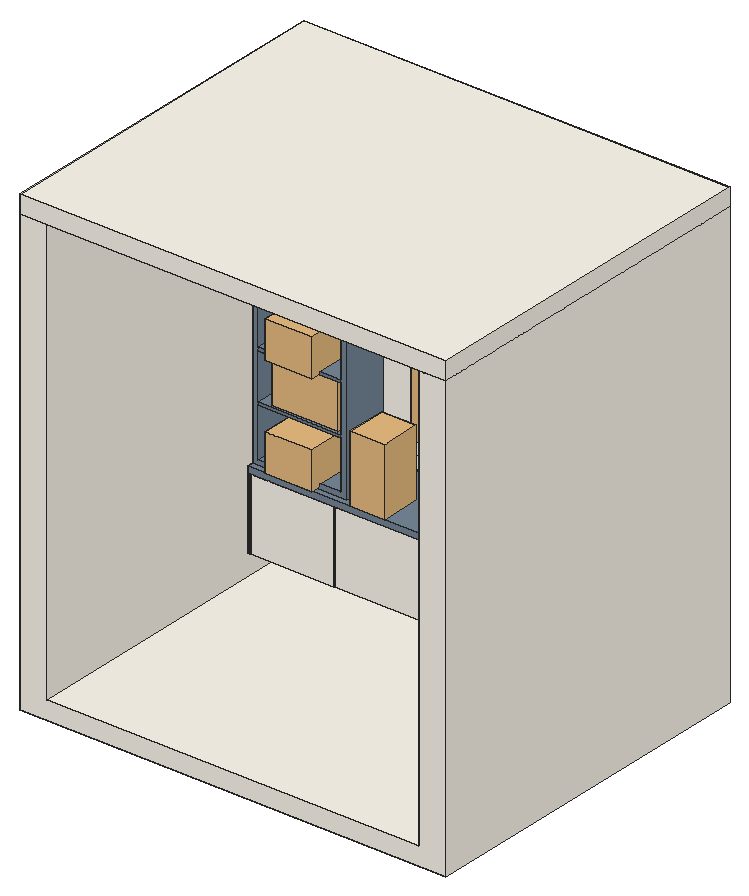
# SketchUp Ruby script. Lengths in inches.
U = 1.inch
M = Sketchup.active_model
def pt(a) = Geom::Point3d.new(a.map { |v| v * U })
def face(e, loops, mat)
  f = e.add_face(loops[0].map { |a| pt(a) })
  loops[1..].each { |l| e.add_face(l.map { |a| pt(a) }).erase! }
  f.material = f.back_material = mat if mat
  f
end
# faces: each face lists its corners as indices into pts; further lists are holes
def faces(e, pts, list, mat = nil) = list.each { |f| face(e, (f[0].is_a?(Array) ? f : [f]).map { |l| l.map { |i| pts[i] } }, mat) }
# xy, xz, yz: faces in a plane at the given z, y or x. An outline is a flat list of corners, or four numbers for a rectangle; further outlines are holes
def ring(l) = l.size == 4 ? [[l[0], l[1]], [l[2], l[1]], [l[2], l[3]], [l[0], l[3]]] : l.each_slice(2).to_a
def flat(e, list, mat, &to3) = list.each { |f| face(e, (f[0].is_a?(Array) ? f : [f]).map { |l| ring(l).map { |u, v| to3.(u, v) } }, mat) }
def xy(e, z, list, mat = nil) = flat(e, list, mat) { |x, y| [x, y, z] }
def xz(e, y, list, mat = nil) = flat(e, list, mat) { |x, z| [x, y, z] }
def yz(e, x, list, mat = nil) = flat(e, list, mat) { |y, z| [x, y, z] }
def lines(e, pts, list) = list.each { |a, b| e.add_line(pt(pts[a]), pt(pts[b])) }
# prism: a flat outline (further loops are holes) pulled along v
def prism(e, loops, v, mat = nil)
  f = face(e, loops, mat); d = Geom::Vector3d.new(v.map { |x| x * U })
  f.pushpull(f.normal.samedirection?(d) ? d.length : -d.length)
end
def box(e, o, s, mat = nil) = prism(e, [[o, [o[0] + s[0], o[1], o[2]], [o[0] + s[0], o[1] + s[1], o[2]], [o[0], o[1] + s[1], o[2]]]], [0, 0, s[2]], mat)
def at(x, y, z, deg = 0) = Geom::Transformation.translation(pt([x, y, z])) * Geom::Transformation.rotation(ORIGIN, Z_AXIS, deg.degrees)
def axes(o, x, y, z) = Geom::Transformation.new([*x, 0, *y, 0, *z, 0, *pt(o).to_a, 1])
def part(name) = M.definitions.add(name)
# library, detail: a bought-in or finely detailed component or shape, given as its bounding box
def library(name, o, s) = part(name).tap { |d| box(d.entities, o, s) }
def detail(e, o, s) = box(e.add_group.entities, o, s)
def put(e, d, t, mat = nil) = e.add_instance(d, t).tap { |i| i.material = mat if mat }
def group(e, t, mat = nil) = e.add_group.tap { |g| g.transformation = t; g.material = mat if mat }.entities
root = M.entities
M.materials.add("[0052_FloralWhite]").color = [255, 250, 240]
M.materials.add("[0110_LightSlateGray]").color = [119, 136, 153]
M.materials.add("[0111_SlateGray]").color = [112, 128, 144]
c1 = library("TV (1)",[0,0,0],[57.09,0.98,33.46])
c2 = library("Potted plant",[-1.15,-1.29,0],[7.65,7.78,5.89])
c3 = library("plants",[-0.26,-0.03,0],[11.57,13.37,22.79])
c4 = library("Decorative sailing ship",[0,0,0],[34.02,11.3,29.65])
c5 = library("horse",[-15.44,-5.1,-1.44],[29.35,10.2,27.55])
box(root,[0,0,150],[144,120,6],"[0052_FloralWhite]")
put(root,c1,axes([52.71,99.5,56.52],[1,0,0],[0,2.85,0],[0,0,1]))
put(root,c2,axes([18.09,86.57,40.3],[2.08,0,0],[0,2.0976,0],[0,0,2.12906]))
put(root,c2,axes([18.09,86.57,107],[2.08,0,0],[0,2.0976,0],[0,0,2.12906]))
put(root,c2,axes([18.09,86.57,74.48],[2.08,0,0],[0,2.0976,0],[0,0,2.12906]))
put(root,c2,axes([103.27,88.1875,113.32],[2.08,0,0],[0,2.0976,0],[0,0,2.12906]))
put(root,c2,axes([44.71,88.1875,113.32],[2.08,0,0],[0,2.0976,0],[0,0,2.12906]))
put(root,c3,at(43.99,85,39.5625))
put(root,c4,axes([10.82,82.23,91.875],[0.7885,0,0],[0,1.67,0],[0,0,0.5025]))
put(root,c5,axes([26.54,96.08,58.2],[0.7654,0,0],[0,1.59,0],[0,0,0.61717]))
g1 = group(root,at(0,0,0))
xy(g1,0,[[0,0,144,120]])
xy(g1,6,[[9,0,135,0,135,109,132.6,109,132.6,111,130.2,111,130.2,109,127.8,109,127.8,111,125.4,111,125.4,109,123,109,123,111,120.6,111,120.6,109,118.2,109,118.2,111,115.8,111,115.8,109,113.4,109,113.4,111,111,111,111,109,108.6,109,108.6,111,106.2,111,106.2,109,103.8,109,103.8,111,101.4,111,101.4,109,99,109,99,111,9,111]],"[0052_FloralWhite]")
xy(g1,13.1875,[[9,85,9,111,99,111,99,109,125.1875,109,125.1875,85,124.33,85,124.33,89.0625,124.13,89.0625,124.13,85,95.68,85,95.68,89.0625,95.48,89.0625,95.48,85,67.02,85,67.02,89.0625,66.82,89.0625,66.82,85,38.37,85,38.37,89.0625,38.17,89.0625,38.17,85,9.91,85,9.91,89.0625,9.71,89.0625,9.71,85]],"[0052_FloralWhite]")
xy(g1,37.36,[[9.91,85,38.17,85,38.17,89.0625,38.37,89.0625,38.37,85,66.82,85,66.82,89.0625,67.02,89.0625,67.02,85,95.48,85,95.48,89.0625,95.68,89.0625,95.68,85,124.13,85,124.13,89.0625,124.33,89.0625,124.33,90,9.71,90,9.71,89.0625,9.91,89.0625]])
xy(g1,37.5625,[[9.71,85,124.33,90]])
xy(g1,39.5625,[[9,85,125.1875,85,125.1875,109,99,109,99,111,40.875,111,40.875,87,9,87]],"[0110_LightSlateGray]")
xy(g1,41.1875,[[11,87,38.875,111]],"[0110_LightSlateGray]")
xy(g1,50.4375,[[40.875,102.3,125.1875,103.11]])
xy(g1,57.75,[[11,87,38.875,111]],"[0110_LightSlateGray]")
xy(g1,58.75,[[11,87,38.875,111]],"[0110_LightSlateGray]")
xy(g1,74.3125,[[11,87,38.875,111]],"[0110_LightSlateGray]")
xy(g1,75.3125,[[11,87,38.875,111]],"[0110_LightSlateGray]")
xy(g1,90.875,[[11,87,38.875,111]],"[0110_LightSlateGray]")
xy(g1,91.875,[[11,87,38.875,111]],"[0110_LightSlateGray]")
xy(g1,95.5625,[[40.875,102.3,125.1875,103.11]],"[0052_FloralWhite]")
xy(g1,107.4375,[[11,87,38.875,111]],"[0110_LightSlateGray]")
xy(g1,108.4375,[[11,87,38.875,111]],"[0110_LightSlateGray]")
xy(g1,113.59,[[40.875,87,40.875,111,99,111,99,109,125.1875,109,125.1875,87]],"[0110_LightSlateGray]")
xy(g1,114.73,[[40.875,87,125.1875,87,125.1875,109,99,109,99,111,40.875,111]],"[0110_LightSlateGray]")
xy(g1,124,[[11,87,38.875,111]],"[0111_SlateGray]")
xy(g1,126,[[9,87,40.875,111],[99,109,101.4,111],[103.8,109,106.2,111],[108.6,109,111,111],[113.4,109,115.8,111],
  [118.2,109,120.6,111],[123,109,125.4,111],[127.8,109,130.2,111],[132.6,109,135,111]],"[0110_LightSlateGray]")
xy(g1,137.05,[[0,105,9,111],[135,105,144,111]])
xy(g1,137.05,[[9,105,135,111]],"[0052_FloralWhite]")
xy(g1,150,[[0,0,9,105],[135,0,144,105]],"[0052_FloralWhite]")
xy(g1,150,[[0,105,144,120]],"[0110_LightSlateGray]")
xz(g1,0,[[0,0,144,0,144,150,135,150,135,6,9,6,9,150,0,150]],"[0052_FloralWhite]")
xz(g1,85,[[9.91,13.1875,38.17,37.36],[38.37,13.1875,66.82,37.36],[67.02,13.1875,95.48,37.36],[95.68,13.1875,124.13,37.36]],"[0052_FloralWhite]")
xz(g1,85,[[9,13.1875,9.71,13.1875,9.71,37.5625,124.33,37.5625,124.33,13.1875,125.1875,13.1875,125.1875,39.5625,9,39.5625]],"[0110_LightSlateGray]")
xz(g1,87,[[[9,39.5625,40.875,39.5625,40.875,113.59,125.1875,113.59,125.1875,114.73,40.875,114.73,40.875,126,9,126],[11,41.1875,38.875,124]],[11,107.4375,38.875,108.4375]],"[0110_LightSlateGray]")
xz(g1,87,[[11,57.75,38.875,58.75],[11,74.3125,38.875,75.3125],[11,90.875,38.875,91.875]],"[0111_SlateGray]")
xz(g1,89.0625,[[9.71,13.1875,9.91,37.36],[38.17,13.1875,38.37,37.36],[66.82,13.1875,67.02,37.36],[95.48,13.1875,95.68,37.36],[124.13,13.1875,124.33,37.36]])
xz(g1,90,[[9.71,37.36,124.33,37.5625]])
xz(g1,102.3,[[40.875,50.4375,125.1875,95.5625]],"[0052_FloralWhite]")
xz(g1,103.11,[[40.875,50.4375,125.1875,95.5625]],"[0052_FloralWhite]")
xz(g1,105,[[0,137.05,9,150],[135,137.05,144,150]])
xz(g1,105,[[9,137.05,135,150]],"[0052_FloralWhite]")
xz(g1,109,[[99,13.1875,101.4,39.5625],[101.4,13.1875,103.8,39.5625],[103.8,13.1875,106.2,39.5625],[106.2,13.1875,108.6,39.5625],[108.6,13.1875,111,39.5625],
  [111,13.1875,113.4,39.5625],[113.4,13.1875,115.8,39.5625],[115.8,13.1875,118.2,39.5625],[118.2,13.1875,120.6,39.5625],[120.6,13.1875,123,39.5625],
  [123,13.1875,125.1875,39.5625],[99,113.59,101.4,114.73],[101.4,113.59,103.8,114.73],[103.8,113.59,106.2,114.73],[106.2,113.59,108.6,114.73],
  [108.6,113.59,111,114.73],[111,113.59,113.4,114.73],[113.4,113.59,115.8,114.73],[115.8,113.59,118.2,114.73],[118.2,113.59,120.6,114.73],
  [120.6,113.59,123,114.73],[123,113.59,125.1875,114.73]])
xz(g1,109,[[99,6,101.4,13.1875],[103.8,6,106.2,13.1875],[108.6,6,111,13.1875],[113.4,6,115.8,13.1875],[118.2,6,120.6,13.1875],
  [123,6,125.4,6,125.4,126,123,126,123,114.73,125.1875,114.73,125.1875,113.59,123,113.59,123,39.5625,125.1875,39.5625,125.1875,13.1875,123,13.1875],[127.8,6,130.2,126],[132.6,6,135,126],[99,39.5625,101.4,113.59],[103.8,39.5625,106.2,113.59],
  [108.6,39.5625,111,113.59],[113.4,39.5625,115.8,113.59],[118.2,39.5625,120.6,113.59],[99,114.73,101.4,126],[103.8,114.73,106.2,126],
  [108.6,114.73,111,126],[113.4,114.73,115.8,126],[118.2,114.73,120.6,126]],"[0110_LightSlateGray]")
xz(g1,111,[[9,6,99,13.1875],[[9,13.1875,99,13.1875,99,39.5625,40.875,39.5625,40.875,113.59,99,113.59,99,114.73,40.875,114.73,40.875,126,9,126],[11,41.1875,38.875,57.75],[11,108.4375,38.875,124],[11,91.875,38.875,107.4375],[11,75.3125,38.875,90.875],[11,58.75,38.875,74.3125]]])
xz(g1,111,[[101.4,6,103.8,6,103.8,126,106.2,126,106.2,6,108.6,6,108.6,126,111,126,111,6,113.4,6,113.4,126,115.8,126,115.8,6,118.2,6,118.2,126,120.6,126,120.6,6,123,6,123,126,125.4,126,125.4,6,127.8,6,127.8,126,130.2,126,130.2,6,132.6,6,132.6,126,135,126,135,137.05,9,137.05,9,126,40.875,126,40.875,114.73,99,114.73,99,126,101.4,126],[40.875,39.5625,99,113.59]],"[0052_FloralWhite]")
xz(g1,111,[[11,41.1875,38.875,57.75],[11,58.75,38.875,74.3125],[11,75.3125,38.875,90.875],[11,91.875,38.875,107.4375],[11,108.4375,38.875,124]],"[0110_LightSlateGray]")
xz(g1,120,[[0,0,144,150]],"[0052_FloralWhite]")
yz(g1,0,[[0,0,120,150]],"[0052_FloralWhite]")
yz(g1,9,[[85,13.1875,111,13.1875,111,126,87,126,87,39.5625,85,39.5625]])
yz(g1,9,[[0,6,111,6,111,13.1875,85,13.1875,85,39.5625,87,39.5625,87,126,111,126,111,137.05,105,137.05,105,150,0,150]],"[0052_FloralWhite]")
yz(g1,9,[[85,13.1875,85,39.5625,87,39.5625,87,126,111,126,111,13.1875]],"[0110_LightSlateGray]")
yz(g1,9.71,[[85,13.1875,89.0625,37.36],[85,37.36,90,37.5625]])
yz(g1,9.91,[[85,13.1875,89.0625,37.36]])
yz(g1,11,[[87,41.1875,111,57.75],[87,58.75,111,74.3125],[87,75.3125,111,90.875],[87,91.875,111,107.4375],[87,108.4375,111,124]],"[0110_LightSlateGray]")
yz(g1,38.17,[[85,13.1875,89.0625,37.36]])
yz(g1,38.37,[[85,13.1875,89.0625,37.36]])
yz(g1,38.875,[[87,41.1875,111,57.75],[87,58.75,111,74.3125],[87,75.3125,111,90.875],[87,91.875,111,107.4375],[87,108.4375,111,124]],"[0110_LightSlateGray]")
yz(g1,40.875,[[[87,39.5625,111,113.59],[102.3,50.4375,103.11,95.5625]],[87,114.73,111,126]],"[0110_LightSlateGray]")
yz(g1,66.82,[[85,13.1875,89.0625,37.36]])
yz(g1,67.02,[[85,13.1875,89.0625,37.36]])
yz(g1,95.48,[[85,13.1875,89.0625,37.36]])
yz(g1,95.68,[[85,13.1875,89.0625,37.36]])
yz(g1,99,[[109,6,111,13.1875],[109,13.1875,111,39.5625],[109,113.59,111,114.73],[109,114.73,111,126]])
yz(g1,99,[[109,39.5625,111,113.59]],"[0110_LightSlateGray]")
yz(g1,101.4,[[109,6,111,126]],"[0110_LightSlateGray]")
yz(g1,103.8,[[109,6,111,126]],"[0110_LightSlateGray]")
yz(g1,106.2,[[109,6,111,126]],"[0110_LightSlateGray]")
yz(g1,108.6,[[109,6,111,126]],"[0110_LightSlateGray]")
yz(g1,111,[[109,6,111,126]],"[0110_LightSlateGray]")
yz(g1,113.4,[[109,6,111,126]],"[0110_LightSlateGray]")
yz(g1,115.8,[[109,6,111,126]],"[0110_LightSlateGray]")
yz(g1,118.2,[[109,6,111,126]],"[0110_LightSlateGray]")
yz(g1,120.6,[[109,6,111,126]],"[0110_LightSlateGray]")
yz(g1,123,[[109,6,111,126]],"[0110_LightSlateGray]")
yz(g1,124.13,[[85,13.1875,89.0625,37.36]])
yz(g1,124.33,[[85,13.1875,89.0625,37.36],[85,37.36,90,37.5625]])
yz(g1,125.1875,[[102.3,50.4375,103.11,95.5625]],"[0052_FloralWhite]")
yz(g1,125.1875,[[85,13.1875,109,39.5625],[87,113.59,109,114.73]],"[0110_LightSlateGray]")
yz(g1,125.4,[[109,6,111,126]],"[0110_LightSlateGray]")
yz(g1,127.8,[[109,6,111,126]],"[0110_LightSlateGray]")
yz(g1,130.2,[[109,6,111,126]],"[0110_LightSlateGray]")
yz(g1,132.6,[[109,6,111,126]],"[0110_LightSlateGray]")
yz(g1,135,[[109,126,111,137.05]])
yz(g1,135,[[0,6,0,150,105,150,105,137.05,109,137.05,109,6]],"[0052_FloralWhite]")
yz(g1,144,[[0,0,120,150]],"[0052_FloralWhite]")
